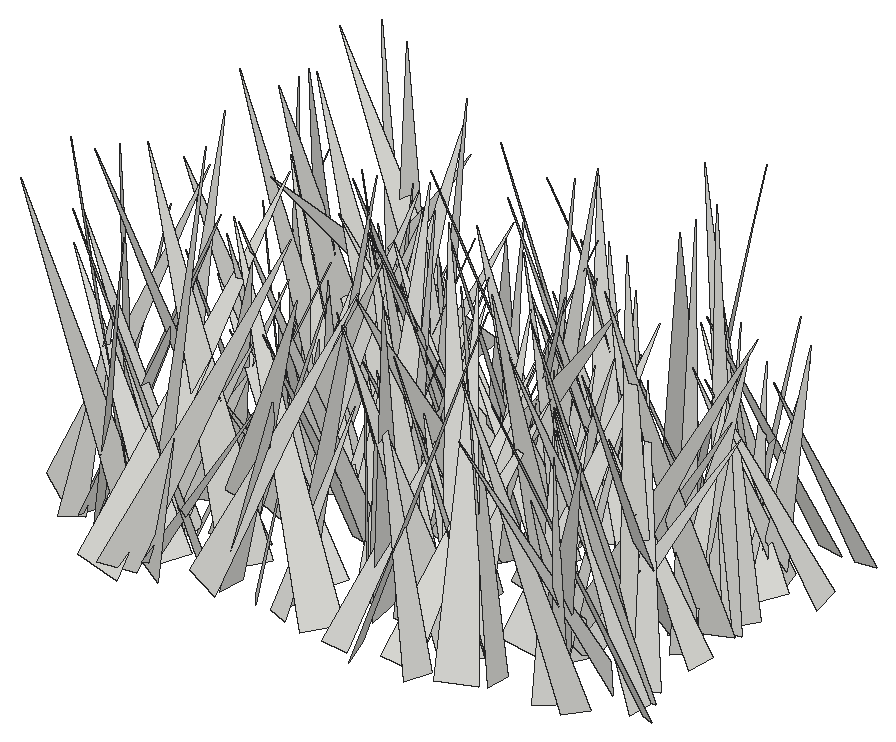
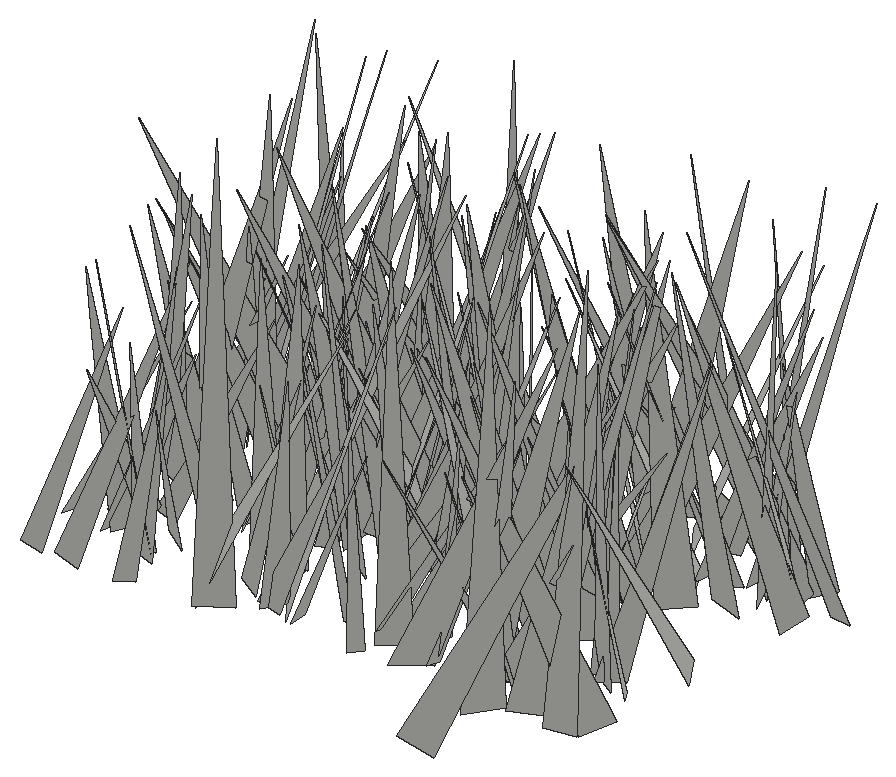
# SketchUp Ruby script. Lengths in inches.
U = 1.inch
M = Sketchup.active_model
def pt(a) = Geom::Point3d.new(a.map { |v| v * U })
def face(e, loops, mat)
  f = e.add_face(loops[0].map { |a| pt(a) })
  loops[1..].each { |l| e.add_face(l.map { |a| pt(a) }).erase! }
  f.material = f.back_material = mat if mat
  f
end
# faces: each face lists its corners as indices into pts; further lists are holes
def faces(e, pts, list, mat = nil) = list.each { |f| face(e, (f[0].is_a?(Array) ? f : [f]).map { |l| l.map { |i| pts[i] } }, mat) }
# xy, xz, yz: faces in a plane at the given z, y or x. An outline is a flat list of corners, or four numbers for a rectangle; further outlines are holes
def ring(l) = l.size == 4 ? [[l[0], l[1]], [l[2], l[1]], [l[2], l[3]], [l[0], l[3]]] : l.each_slice(2).to_a
def flat(e, list, mat, &to3) = list.each { |f| face(e, (f[0].is_a?(Array) ? f : [f]).map { |l| ring(l).map { |u, v| to3.(u, v) } }, mat) }
def xy(e, z, list, mat = nil) = flat(e, list, mat) { |x, y| [x, y, z] }
def xz(e, y, list, mat = nil) = flat(e, list, mat) { |x, z| [x, y, z] }
def yz(e, x, list, mat = nil) = flat(e, list, mat) { |y, z| [x, y, z] }
def lines(e, pts, list) = list.each { |a, b| e.add_line(pt(pts[a]), pt(pts[b])) }
# prism: a flat outline (further loops are holes) pulled along v
def prism(e, loops, v, mat = nil)
  f = face(e, loops, mat); d = Geom::Vector3d.new(v.map { |x| x * U })
  f.pushpull(f.normal.samedirection?(d) ? d.length : -d.length)
end
def box(e, o, s, mat = nil) = prism(e, [[o, [o[0] + s[0], o[1], o[2]], [o[0] + s[0], o[1] + s[1], o[2]], [o[0], o[1] + s[1], o[2]]]], [0, 0, s[2]], mat)
def at(x, y, z, deg = 0) = Geom::Transformation.translation(pt([x, y, z])) * Geom::Transformation.rotation(ORIGIN, Z_AXIS, deg.degrees)
def axes(o, x, y, z) = Geom::Transformation.new([*x, 0, *y, 0, *z, 0, *pt(o).to_a, 1])
def part(name) = M.definitions.add(name)
# library, detail: a bought-in or finely detailed component or shape, given as its bounding box
def library(name, o, s) = part(name).tap { |d| box(d.entities, o, s) }
def detail(e, o, s) = box(e.add_group.entities, o, s)
def put(e, d, t, mat = nil) = e.add_instance(d, t).tap { |i| i.material = mat if mat }
def group(e, t, mat = nil) = e.add_group.tap { |g| g.transformation = t; g.material = mat if mat }.entities
root = M.entities
c1 = part("fur_instance\#9")
p = [[0.8125,0,1.79],[0.67,-0.02,1.48],[0,-0.11,0],[0,0.11,0]]
faces(c1.entities,p,[[0,1,2,3]])
put(root,c1,axes([481.6,86.91,-21.86],[-7.48109,-1.28394,1.71532],[-0.94889,7.57103,1.5286],[1.92105,-1.26035,7.43496]))
put(root,c1,axes([495.89,84.79,-21.86],[-5.54027,1.19429,0.93196],[1.15956,5.61711,-0.30487],[0.97482,0.10593,5.65933]))
put(root,c1,axes([501.27,88.96,-21.86],[-5.37416,-4.85351,0.14678],[-4.51514,5.07548,2.5125],[1.7865,-1.77274,6.79157]))
put(root,c1,axes([480,86.77,-21.66],[6.17791,2.14602,1.95241],[2.61385,-6.11017,-1.55482],[-1.25898,-2.15507,6.35252]))
put(root,c1,axes([485.14,86.22,-21.86],[-5.86461,-3.9483,0.52207],[-3.9663,5.70596,-1.40208],[-0.36068,1.452,6.92942]))
put(root,c1,axes([498.78,88.76,-21.86],[-0.05965,-7.49908,0.31223],[-6.76708,0.1888,3.24163],[3.24657,0.25574,6.76251]))
put(root,c1,axes([493.06,84.84,-21.86],[6.96857,2.87265,0.80723],[2.85827,-7.01507,0.2896],[-0.85676,-0.03815,7.53188]))
put(root,c1,axes([502.04,86.01,-21.66],[-0.7555,-5.85213,2.53673],[-5.87032,-0.36099,-2.58111],[-2.49433,2.62211,5.30623]))
put(root,c1,axes([495.42,87.4375,-21.86],[-6.6748,0.96554,1.83268],[1.43583,6.61336,1.7452],[1.49311,-2.0433,6.51456]))
put(root,c1,axes([483.82,84.82,-21.86],[4.31651,6.80061,2.35568],[7.01576,-4.58865,0.3914],[-1.60519,-1.76799,8.04533]))
put(root,c1,axes([501,86.47,-21.86],[-1.48378,-4.80354,1.85374],[-5.06695,1.70492,0.36217],[0.91449,1.65264,5.01442]))
put(root,c1,axes([492.03,88.03,-21.86],[7.80174,-0.94154,1.76979],[-0.49694,-7.7978,-1.95786],[-1.94209,-1.78708,7.61055]))
put(root,c1,axes([482.92,84.07,-21.66],[6.18283,-3.26103,2.17206],[-3.91127,-5.37775,3.05962],[-0.2327,3.74499,6.28493]))
put(root,c1,axes([486.67,85.82,-21.86],[5.61379,-0.0924,1.25595],[-0.17391,-5.73971,0.3551],[-1.24727,0.38445,5.60331]))
put(root,c1,axes([487.98,85.58,-21.86],[-2.4957,-1.61977,2.11338],[-2.18018,2.90599,-0.34732],[1.52869,1.50005,2.95492]))
put(root,c1,axes([481.2,87.21,-21.86],[-5.20637,-5.83633,2.28098],[-6.06397,5.44004,0.07832],[1.57922,1.64775,7.82067]))
put(root,c1,axes([484.88,88.07,-21.66],[3.43044,-6.71204,0.2285],[-6.5076,-3.25868,1.97581],[1.6598,1.09595,7.27431]))
put(root,c1,axes([483.93,86.05,-21.86],[-4.33384,4.15795,0.46311],[4.09626,4.08164,1.68703],[-0.85069,-1.52868,5.76409]))
put(root,c1,axes([479.18,86.21,-21.86],[3.46953,-2.67132,1.40146],[-2.94376,-3.4648,0.68347],[-0.65905,1.41311,4.3251]))
put(root,c1,axes([486.01,85.03,-21.66],[1.82211,6.46965,0.85286],[6.26515,-1.48669,-2.10749],[1.8253,-1.35544,6.38239]))
put(root,c1,axes([504.28,87.23,-21.66],[-3.99389,-5.07881,0.29207],[-4.86869,3.70838,-2.09153],[-1.47493,1.51142,6.11318]))
put(root,c1,axes([489.29,85.17,-21.86],[1.39427,3.92432,0.17719],[3.92808,-1.39069,-0.10895],[0.04345,-0.20342,4.16322]))
put(root,c1,axes([483.59,85.01,-21.66],[3.8069,0.05751,0.20355],[-0.0416,-3.39391,1.73693],[-0.20739,1.73647,3.38805]))
put(root,c1,axes([491.09,85.42,-21.86],[-3.57557,6.64036,0.56629],[6.42877,3.26724,2.27945],[-1.75672,-1.55901,7.1891]))
put(root,c1,axes([497.24,85.27,-21.86],[-2.95766,6.66869,1.17233],[6.76114,2.97762,0.11972],[0.36439,-1.12067,7.29416]))
put(root,c1,axes([482.18,83.92,-21.86],[0.04279,8.23701,0.26485],[7.98617,0.02394,-2.03491],[2.0346,-0.26721,7.98181]))
put(root,c1,axes([486.22,87.3,-21.86],[-5.61004,5.72169,2.32507],[6.16954,5.3361,1.75473],[0.28367,-2.89906,7.81865]))
put(root,c1,axes([496.71,87.7,-21.86],[-5.00716,-3.11226,0.75462],[-3.18598,4.98296,-0.58898],[0.32424,0.90067,5.86608]))
put(root,c1,axes([498.32,86.27,-21.86],[-7.03444,-1.19576,1.59787],[-1.52444,6.99776,-1.47438],[1.28808,1.75153,6.98136]))
put(root,c1,axes([483.23,87.79,-21.86],[-6.42244,0.41118,0.57395],[0.45958,6.42194,0.54196],[0.53597,-0.57954,6.41273]))
put(root,c1,axes([492.22,84.69,-21.86],[-3.33289,3.23483,0.32122],[2.5841,2.91556,-2.549],[1.97223,1.64647,3.88264]))
put(root,c1,axes([503.16,88.4375,-21.86],[-1.48365,-5.76059,1.44193],[-5.8771,1.21156,-1.20691],[-0.85046,1.67706,5.82486]))
put(root,c1,axes([494.95,84.83,-21.66],[-2.16647,5.60636,0.16983],[5.26617,2.09582,-2.00715],[1.93067,0.57445,5.66535]))
put(root,c1,axes([490.73,88.4375,-21.86],[3.47548,2.68418,2.07766],[3.24177,-3.50628,-0.89294],[-1.00618,-2.02524,4.29959]))
put(root,c1,axes([481.95,87.7,-21.86],[2.31497,4.33574,1.17317],[4.28428,-1.73503,-2.04175],[1.34907,-1.93005,4.47091]))
put(root,c1,axes([503.47,87.96,-21.86],[-5.40823,0.65228,0.52882],[0.69912,5.40686,0.48075],[0.46513,-0.5426,5.42617]))
put(root,c1,axes([491.42,87.84,-21.86],[-2.0645,-2.99831,1.70133],[-3.28642,2.31061,0.08412],[1.04107,1.34824,3.63936]))
put(root,c1,axes([500.58,86.02,-21.86],[-4.64664,1.60589,0.29185],[1.45378,4.47236,-1.46283],[0.74202,1.29401,4.69365]))
put(root,c1,axes([479.47,86.95,-21.86],[6.02676,-0.13267,0.65935],[-0.25057,-5.95995,1.09109],[-0.62414,1.1116,5.92866]))
put(root,c1,axes([499.28,89.35,-21.86],[2.57242,-3.23839,0.522],[-3.12857,-2.6216,-0.84629],[-0.98573,-0.13048,4.04824]))
put(root,c1,axes([480.83,87.65,-21.86],[-6.27895,-2.5321,2.5957],[-2.9165,6.61067,-0.60625],[2.15482,1.56906,6.74309]))
put(root,c1,axes([500.79,91.05,-21.86],[-6.83559,-3.49227,1.59422],[-2.83471,6.78714,2.71329],[2.5888,-1.7893,7.18049]))
put(root,c1,axes([495.28,88.22,-21.86],[-3.28307,2.60382,1.30489],[2.8552,3.26547,0.66758],[0.57484,-1.34832,4.13676]))
put(root,c1,axes([485.5,88.91,-21.86],[-3.35024,-7.10363,1.41562],[-6.97339,2.74138,-2.74705],[-1.95891,2.39017,7.35795]))
put(root,c1,axes([477.58,87.37,-21.86],[3.97232,6.71602,1.21655],[6.692,-3.55551,-2.22255],[1.34242,-2.14887,7.47961]))
put(root,c1,axes([489.41,88.01,-21.86],[-4.10469,4.34568,0.4298],[4.19686,3.76273,2.03626],[-1.20665,-1.6956,5.62024]))
put(root,c1,axes([482.57,87.71,-21.86],[3.62784,4.7769,0.79864],[4.78599,-3.38301,-1.50576],[0.74217,-1.53438,5.80626]))
put(root,c1,axes([485.07,88.8125,-21.86],[5.29628,3.42643,1.15131],[3.61426,-4.98862,-1.7797],[0.0553,-2.11891,6.05175]))
put(root,c1,axes([496.3,86.92,-21.86],[-3.06885,7.2619,1.47031],[7.40414,2.94663,0.90053],[-0.27521,-1.70206,7.83212]))
put(root,c1,axes([482.66,90.24,-21.86],[3.94338,-5.9757,0.15667],[-5.94055,-3.89659,0.90015],[0.66588,0.62564,7.10275]))
put(root,c1,axes([495.98,88.3125,-21.86],[-4.03311,-0.04964,1.55556],[-0.10181,4.31995,-0.1261],[1.55302,0.15428,4.03144]))
put(root,c1,axes([494.17,86.58,-21.66],[-1.05033,5.0969,0.69056],[4.61293,1.24522,-2.17458],[2.27512,-0.17172,4.72788]))
put(root,c1,axes([479.54,87.17,-21.86],[-3.93965,-2.75758,3.63418],[-3.8658,4.56754,-0.72493],[2.42222,2.80458,4.7539]))
put(root,c1,axes([489.33,86.24,-21.86],[-7.34355,0.30763,3.29021],[-0.75169,7.65215,-2.39318],[3.21793,2.48952,6.94946]))
put(root,c1,axes([501.06,90.91,-21.86],[-5.87389,-5.06073,1.31002],[-4.91563,6.01764,1.20596],[1.77871,-0.08191,7.65893]))
put(root,c1,axes([501.11,92.44,-21.66],[-2.73458,-7.67612,0.26637],[-7.34259,2.69559,2.30041],[2.25392,-0.53168,7.81722]))
put(root,c1,axes([478.64,88.625,-21.86],[6.73911,-0.51973,0.37006],[-0.5475,-6.72675,0.52311],[-0.32757,0.55072,6.73884]))
put(root,c1,axes([488.04,89.2,-21.86],[1.13242,-3.28388,1.61058],[-3.44754,-1.52145,-0.67814],[-1.2216,1.24962,3.40681]))
put(root,c1,axes([493.41,88.5625,-21.86],[-2.35431,6.5098,1.98677],[6.74258,1.94391,1.62058],[-0.92858,-2.38982,6.73008]))
put(root,c1,axes([488.35,91.19,-21.86],[-1.09873,-5.30096,0.04279],[-5.29764,1.09638,-0.20521],[-0.19227,0.08352,5.40974]))
put(root,c1,axes([483.35,88.11,-21.86],[5.4364,3.24485,0.19999],[3.25087,-5.4295,-0.27539],[-0.03035,-0.33899,6.32516]))
put(root,c1,axes([492.64,88.92,-21.66],[-4.27144,-3.27285,0.83505],[-3.36103,3.98484,-1.57435],[-0.33515,1.75031,5.14569]))
put(root,c1,axes([486.59,90.29,-21.86],[0.42808,-6.23217,1.75974],[-6.34467,-0.7568,-1.13683],[-1.29687,1.64535,6.14254]))
put(root,c1,axes([493.46,93.06,-21.66],[3.75973,-6.87339,0.18092],[-6.4988,-3.61971,-2.46477],[-2.2454,-1.03249,7.43666]))
put(root,c1,axes([484.69,91.89,-21.66],[-2.93741,-3.09466,0.01129],[-2.71699,2.58635,2.03327],[1.48156,-1.39259,3.75115]))
put(root,c1,axes([490.29,90.08,-21.86],[-2.1287,-6.56011,1.58213],[-6.38568,1.42177,-2.69649],[-2.18201,2.23898,6.34786]))
put(root,c1,axes([497.03,91.3,-21.86],[0.47812,-7.3143,1.47747],[-7.45136,-0.54714,-0.29732],[-0.39895,1.45332,7.32388]))
put(root,c1,axes([484.38,90.89,-21.86],[1.4912,-7.63112,1.5604],[-7.07021,-0.65953,3.53123],[3.26816,2.05513,6.92734]))
put(root,c1,axes([493.02,87.54,-21.86],[3.07038,6.62387,1.59445],[6.28566,-3.42873,2.13997],[-2.62838,-0.46188,6.98022]))
put(root,c1,axes([495.49,88.25,-21.66],[-4.4871,3.83069,1.41429],[3.5666,4.69982,-1.41404],[1.98841,0.2144,5.72789]))
put(root,c1,axes([489.61,90.96,-21.86],[6.19787,3.91116,1.13836],[4.069,-5.84754,-2.06304],[0.19042,-2.34857,7.0324]))
put(root,c1,axes([491.51,90.55,-21.86],[-5.53788,-5.2946,2.37412],[-5.70348,5.57065,-0.88067],[1.06751,2.29618,7.61087]))
put(root,c1,axes([486.34,89.77,-21.66],[3.70498,4.05955,2.96614],[3.93602,-4.63444,1.42637],[-3.1282,-1.02317,5.30776]))
put(root,c1,axes([481.3,89.16,-21.86],[1.99412,7.08431,1.8343],[7.27705,-2.12036,0.27805],[-0.77249,-1.68678,7.35436]))
put(root,c1,axes([503.06,88.7,-21.66],[-0.43332,5.55714,0.38235],[5.39105,0.32188,1.43136],[-1.40165,-0.47995,5.3871]))
put(root,c1,axes([487.06,90.49,-21.66],[-2.6027,-3.00196,0.39616],[-2.70686,2.07255,-2.07851],[-1.35707,1.62343,3.38609]))
put(root,c1,axes([501.82,89.85,-21.86],[-0.81741,7.52572,2.31704],[7.8363,0.54876,0.98214],[-0.77303,-2.39493,7.506]))
put(root,c1,axes([499.68,88,-21.66],[2.78013,5.13783,0.11647],[4.85085,-2.66723,1.86951],[-1.69707,0.79284,5.53456]))
put(root,c1,axes([499.58,89.84,-21.66],[2.70061,4.81345,0.08968],[4.52857,-2.505,-1.92033],[1.63383,-1.01307,5.17446]))
put(root,c1,axes([490.61,89.34,-21.86],[-2.23719,7.0676,1.63885],[7.20712,2.3619,-0.34736],[0.83319,-1.45336,7.40509]))
put(root,c1,axes([497.3,88.7,-21.86],[-1.51128,6.4389,0.97646],[6.11666,1.74753,-2.05657],[2.23592,-0.42848,6.28601]))
put(root,c1,axes([502.22,89.88,-21.86],[-4.46035,-2.40279,1.6408],[-2.85913,4.17643,-1.65628],[0.53948,2.26814,4.788]))
put(root,c1,axes([483.2,92.42,-21.86],[-2.16973,-4.86696,0.63571],[-4.9077,2.16207,-0.19771],[0.07681,0.6613,5.32503]))
put(root,c1,axes([499.56,89.24,-21.86],[-7.36083,-0.13148,0.37404],[-0.23398,7.05478,-2.12469],[0.32007,2.13349,7.04874]))
put(root,c1,axes([497.98,89.49,-21.86],[-2.69846,2.82224,0.09608],[2.72603,2.63813,-0.93001],[0.73688,0.57546,3.79233]))
put(root,c1,axes([503.09,91.73,-21.86],[-4.33776,1.46199,0.55548],[1.55819,4.18055,1.16497],[0.13425,-1.28363,4.42678]))
put(root,c1,axes([492.29,93.375,-21.86],[-5.41835,-3.58553,1.38238],[-3.2455,5.54933,1.6725],[2.0576,-0.68883,6.27832]))
put(root,c1,axes([492.27,94.9,-21.66],[-6.0329,-5.73941,0.68236],[-5.34499,5.91535,2.49841],[2.19943,-1.36753,7.94322]))
put(root,c1,axes([487.82,92.63,-21.66],[5.19096,1.17327,0.15724],[1.14991,-4.82989,-1.92283],[0.28108,-1.90867,4.96239]))
put(root,c1,axes([498.68,90.24,-21.66],[6.56364,-3.25708,1.01889],[-3.38805,-5.95385,2.79299],[0.40967,2.94467,6.77415]))
put(root,c1,axes([494.46,91.16,-21.86],[-3.43885,-1.25141,0.28396],[-1.28081,3.29756,-0.97876],[-0.07859,1.01608,3.52615]))
put(root,c1,axes([483.93,91.53,-21.86],[3.27603,2.91205,0.73309],[2.99826,-3.11162,-1.03833],[0.1671,-1.26001,4.25844]))
put(root,c1,axes([494.68,92.12,-21.86],[0.8957,-3.44027,0.95903],[-3.38159,-0.49886,1.36875],[1.14894,1.21373,3.28089]))
put(root,c1,axes([492,93.84,-21.66],[-3.24466,-1.65637,0.06319],[-1.44148,2.88818,1.68993],[0.81834,-1.47993,3.2273]))
put(root,c1,axes([502.38,93.41,-21.66],[0.14854,-7.36709,1.66817],[-7.40985,-0.46607,-1.39849],[-1.46661,1.60862,7.23466]))
put(root,c1,axes([492.3,92.89,-21.66],[1.15805,-3.96128,0.43832],[-3.70743,-0.90324,1.63219],[1.46246,0.84697,3.79062]))
put(root,c1,axes([495.09,93.5,-21.86],[-3.74984,-6.28849,1.24601],[-6.40364,3.74219,-0.38514],[0.30173,1.26879,7.3115]))
put(root,c1,axes([496.51,92.26,-21.86],[-4.30239,2.31555,0.00735],[2.25428,4.18495,1.12996],[-0.52922,-0.99839,4.75348]))
put(root,c1,axes([490.18,93.12,-21.86],[4.31656,-7.06636,0.27005],[-6.24466,-3.6606,4.0303],[3.31821,2.3034,7.23345]))
put(root,c1,axes([498.3,92.22,-21.86],[4.90095,-2.69617,0.00541],[-2.57457,-4.67657,1.67032],[0.80058,1.46597,5.33842]))
put(root,c1,axes([495.54,92.51,-21.86],[2.79577,3.11606,1.7882],[3.42019,-3.00212,-0.11591],[-1.09992,-1.41467,4.18482]))
put(root,c1,axes([492.37,91.15,-21.86],[3.37937,2.22818,0.23171],[2.15143,-3.34494,0.78826],[-0.62436,0.53406,3.97033]))
put(root,c1,axes([490.51,90.8,-21.86],[-0.0626,5.05917,0.30688],[5.04763,0.09003,-0.45456],[0.45914,-0.29998,5.03909]))
put(root,c1,axes([492.65,93.74,-21.86],[6.84395,0.46131,0.76105],[0.6015,-6.74756,-1.31919],[-0.65589,-1.3745,6.73144]))
put(root,c1,axes([489.65,93.23,-21.86],[5.36084,-0.19835,3.29768],[0.06393,-6.27827,-0.48156],[-3.30302,-0.44345,5.34285]))
put(root,c1,axes([483.56,93.9,-21.86],[1.83451,-3.56347,0.05806],[-3.52397,-1.80394,0.62811],[0.53227,0.33851,3.95843]))
put(root,c1,axes([482.54,94.04,-21.86],[-0.97115,-4.17934,0.95629],[-4.09852,1.19278,1.05068],[1.25838,0.65947,4.16006]))
put(root,c1,axes([495.01,93.85,-21.66],[4.68158,-4.31782,3.21331],[-4.18207,-5.59908,-1.43065],[-3.3881,0.94493,6.20597]))
put(root,c1,axes([494.79,94.77,-21.66],[4.08531,-1.79648,1.28746],[-1.24322,-4.1049,-1.78292],[-1.82737,-1.22355,4.09124]))
put(root,c1,axes([491.63,94.3,-21.86],[-2.75065,-6.97463,1.22589],[-6.99898,2.47729,-1.60986],[-1.07823,1.71227,7.32256]))
put(root,c1,axes([489.38,94.33,-21.86],[-0.13278,-3.81265,0.23397],[-3.74221,0.08288,-0.77308],[-0.76609,0.25594,3.73581]))
put(root,c1,axes([494.83,93.55,-21.86],[4.10289,-2.86128,0.97197],[-3.01034,-4.01302,0.89377],[-0.2636,1.29386,4.92156]))
put(root,c1,axes([496.3125,94.58,-21.86],[-5.74525,-5.95088,0.61636],[-5.93253,5.55629,-1.65334],[-0.77329,1.58601,8.10478]))
put(root,c1,axes([484.39,92.54,-21.66],[0.24671,6.36494,1.6516],[6.30189,0.24313,-1.87833],[1.87786,-1.65213,6.08648]))
put(root,c1,axes([496.76,94.37,-21.86],[-3.60372,1.36671,1.25031],[1.68423,3.55609,0.96723],[0.77106,-1.37995,3.73084]))
put(root,c1,axes([491.88,93.93,-21.86],[-3.57331,4.48467,0.98446],[4.4978,3.16833,1.89248],[-0.92266,-1.92337,5.41289]))
put(root,c1,axes([481.65,95.95,-21.66],[4.12034,-0.14152,0.59374],[0.17297,-3.61498,-2.06197],[-0.58535,-2.06437,3.57009]))
put(root,c1,axes([481.18,95.8,-21.86],[5.01755,-2.86523,2.69296],[-2.1597,-5.65647,-1.99435],[-3.28592,-0.6574,5.42291]))
put(root,c1,axes([498.92,93.48,-21.86],[-1.92431,3.57441,0.40694],[3.46774,1.72017,1.28872],[-0.95749,-0.95373,3.84949]))
put(root,c1,axes([501.4,92.69,-21.86],[-0.62067,4.74172,0.56344],[4.77083,0.63973,-0.12835],[0.20124,-0.5417,4.78044]))
put(root,c1,axes([492.55,93.4,-21.86],[1.055,3.81063,1.04337],[3.83467,-1.24762,0.6792],[-0.95124,-0.80317,3.89521]))
put(root,c1,axes([487.48,92.42,-21.66],[-4.32625,3.6169,1.13686],[3.35652,4.45591,-1.40339],[1.76301,0.39209,5.46158]))
put(root,c1,axes([491.28,92.08,-21.86],[5.73522,3.47371,0.17785],[3.39582,-5.66618,1.16354],[-0.75282,0.90483,6.60345]))
put(root,c1,axes([483.65,92.77,-21.86],[-0.33332,4.6985,0.41104],[4.65173,0.39553,-0.74898],[0.77866,-0.35159,4.65038]))
put(root,c1,axes([498.14,94.76,-21.86],[3.40491,-1.73217,0.1961],[-1.74293,-3.39081,0.31125],[-0.03288,0.3664,3.80749]))
put(root,c1,axes([497.35,95.47,-21.86],[-6.81995,-3.62088,0.84533],[-3.65528,6.85252,-0.13797],[0.68141,0.51893,7.72033]))
put(root,c1,axes([493.19,92.6,-21.66],[-6.05732,0.47074,1.68041],[-0.07648,5.99257,-1.95441],[1.74342,1.89841,5.75265]))
put(root,c1,axes([498.39,94.84,-21.86],[-4.80301,-2.64529,0.12183],[-2.62964,4.73476,-0.865],[-0.31202,0.81591,5.41463]))
put(root,c1,axes([484.19,95.35,-21.86],[-7.83608,-0.63477,1.59162],[-0.4911,7.96997,0.76075],[1.64165,-0.64574,7.82485]))
put(root,c1,axes([500.04,94.45,-21.86],[-1.7832,4.7887,2.83203],[5.02838,2.65983,-1.33139],[2.38064,-2.03113,4.93345]))
put(root,c1,axes([489.93,92.92,-21.66],[3.45024,7.01244,2.07893],[6.95776,-3.8555,1.45774],[-2.25516,-1.1667,7.67811]))
put(root,c1,axes([502.15,91.92,-21.86],[-7.67594,0.43258,1.18162],[-0.05572,7.18028,-2.99063],[1.25708,2.9597,7.0826]))
put(root,c1,axes([495.43,93.18,-21.86],[0.25291,3.93977,0.05992],[3.89833,-0.25892,0.57035],[-0.57304,-0.02262,3.90646]))
put(root,c1,axes([500.79,96.28,-21.86],[-0.19761,-4.29399,0.26182],[-4.09062,0.10641,-1.34218],[-1.33181,0.31028,4.08362]))
put(root,c1,axes([482.98,96.15,-21.86],[0.8236,-4.35079,0.44599],[-4.32851,-0.74586,0.71716],[0.62636,0.56649,4.3696]))
put(root,c1,axes([485.59,93.5,-21.86],[-1.50811,5.89701,0.63499],[5.61901,1.21081,2.10069],[-1.89858,-1.1007,5.71281]))
put(root,c1,axes([489.25,95.24,-21.86],[-4.02078,2.93374,1.78068],[3.22926,4.16274,0.43339],[1.1617,-1.41743,4.95839]))
put(root,c1,axes([485.93,95.59,-21.86],[3.66443,-1.25509,0.51627],[-1.25966,-3.69872,-0.05095],[-0.50503,0.11865,3.87307]))
put(root,c1,axes([494.21,93.52,-21.66],[-6.74927,1.80081,2.69667],[1.18797,7.16726,-1.81295],[3.01723,1.2063,6.74602]))
put(root,c1,axes([486.32,93.76,-21.86],[-1.25446,7.26591,1.58891],[7.27727,1.53186,-1.25954],[1.53602,-1.32352,7.26503]))
put(root,c1,axes([496.72,95.68,-21.86],[4.30224,-3.16543,2.15858],[-3.43037,-4.62804,0.05027],[-1.70646,1.32286,5.34104]))
put(root,c1,axes([489.27,96.91,-21.86],[-5.99784,0.36822,0.31916],[0.44096,5.77868,1.61988],[0.20737,-1.63795,5.78668]))
put(root,c1,axes([502.34,94.03,-21.86],[0.70044,7.59304,1.85976],[7.56257,-1.13109,1.76971],[-1.98005,-1.63401,7.41708]))
put(root,c1,axes([485.41,94.72,-21.86],[3.56009,0.21869,0.65734],[0.01468,-3.46445,1.07311],[-0.69261,1.05069,3.40155]))
put(root,c1,axes([493.25,94.92,-21.86],[3.25616,5.95918,2.11371],[6.15078,-3.5363,0.49462],[-1.46542,-1.60155,6.77272]))
put(root,c1,axes([480.08,96.29,-21.86],[3.15545,2.01724,0.79775],[2.15051,-3.09372,-0.68323],[-0.2846,-1.01105,3.6823]))
put(root,c1,axes([479.14,93.78,-21.66],[4.7893,3.01055,0.30481],[2.77693,-4.59952,1.79634],[-1.20208,1.36921,5.36414]))
put(root,c1,axes([485.99,96.61,-21.86],[-6.02527,4.37662,1.94606],[4.73834,5.90349,1.39383],[0.70004,-2.28907,7.31546]))
put(root,c1,axes([488.75,98.49,-21.86],[1.84605,-6.6162,0.27609],[-6.51912,-1.76548,1.28157],[1.16252,0.60597,6.74831]))
put(root,c1,axes([484.09,98.2,-21.86],[6.81977,1.54998,0.06465],[1.44583,-6.24479,-2.79788],[0.56233,-2.74155,6.40965]))
put(root,c1,axes([494.41,96.6,-21.86],[3.27913,1.40298,0.59687],[1.4938,-3.23974,-0.59158],[-0.30522,-0.78299,3.51725]))
put(root,c1,axes([481.4,95.95,-21.86],[3.04497,5.63186,2.55497],[5.93211,-3.46487,0.56775],[-1.7481,-1.94792,6.3771]))
put(root,c1,axes([489.45,98.14,-21.66],[-4.59032,-0.23962,0.17171],[-0.16134,4.28449,1.66587],[0.24672,-1.65642,4.28408]))
put(root,c1,axes([502.66,94.55,-21.66],[-8.1921,1.36867,0.61461],[1.20152,8.02801,-1.8625],[0.89853,1.74336,8.09413]))
put(root,c1,axes([503.6875,98,-21.86],[-4.90231,-0.23018,0.15933],[-0.18525,4.76264,1.18065],[0.20988,-1.17272,4.76358]))
put(root,c1,axes([501.85,98.21,-21.86],[-4.7933,-0.97536,0.74224],[-0.77682,4.73507,1.20565],[0.94805,-1.05153,4.74061]))
put(root,c1,axes([487.96,96.71,-21.86],[-4.49863,-0.46507,1.40367],[-0.60193,4.68178,-0.37796],[1.35065,0.53749,4.50678]))
put(root,c1,axes([482.48,97.14,-21.66],[0.05129,-4.93553,2.34933],[-4.99892,0.90807,2.01684],[2.21125,2.16734,4.50493]))
put(root,c1,axes([481.99,99.34,-21.86],[5.20163,-5.29224,1.8402],[-4.95757,-5.51713,-1.85336],[-2.61089,-0.0677,7.18539]))
put(root,c1,axes([486.84,98.66,-21.86],[-4.25051,-1.02119,0.70994],[-0.79222,4.17184,1.25768],[0.95876,-1.08007,4.18663]))
put(root,c1,axes([480.32,99.7,-21.86],[-1.25565,-8.18969,1.33935],[-8.04493,1.53362,1.83538],[2.03567,1.00923,8.07955]))
put(root,c1,axes([495.2,96.46,-21.86],[-2.95923,6.17255,1.7602],[6.41346,2.92118,0.53848],[0.25723,-1.82266,6.82403]))
put(root,c1,axes([495.2,100.5625,-21.66],[1.43301,-8.2393,0.15598],[-8.02359,-1.35888,1.93375],[1.87948,0.48092,8.13635]))
put(root,c1,axes([495.32,98.43,-21.86],[-2.87551,-4.98025,1.4124],[-5.17006,2.84441,-0.49611],[0.26119,1.47404,5.72934]))
put(root,c1,axes([490.94,98.26,-21.86],[3.06956,3.90435,1.71137],[4.25532,-2.68017,-1.51785],[0.25498,-2.27325,4.72887]))
put(root,c1,axes([502.1,97.05,-21.86],[-3.00277,4.1066,0.06153],[3.92812,2.84936,1.52829],[-1.19912,-0.94951,4.85234]))
put(root,c1,axes([501.38,97.77,-21.86],[4.20018,-2.603,1.54886],[-2.85846,-4.28223,0.55487],[-1.0019,1.30501,4.91012]))
put(root,c1,axes([484.49,97.3,-21.86],[4.52412,1.43506,1.852],[1.32361,-4.8885,0.5546],[-1.93323,0.01133,4.71375]))
put(root,c1,axes([484.22,98.03,-21.86],[-2.52559,2.65872,0.46687],[2.62617,2.27215,1.26725],[-0.62447,-1.19747,3.44114]))
put(root,c1,axes([487.69,97.17,-21.86],[-3.44021,1.49763,0.22694],[1.46636,3.43395,-0.43273],[0.37973,0.30751,3.72702]))
put(root,c1,axes([489.3,99.95,-21.66],[-0.15941,-4.26775,0.08772],[-3.87813,0.18147,1.78158],[1.78369,0.01316,3.88138]))
put(root,c1,axes([499.67,99.02,-21.86],[-1.75963,-5.21212,1.71135],[-5.46295,1.82898,-0.04671],[0.50104,1.63703,5.50093]))
put(root,c1,axes([493.37,98.75,-21.86],[-5.74367,-4.09689,1.01684],[-4.21686,5.6466,-1.0688],[0.19121,1.46278,6.97366]))
put(root,c1,axes([501.24,96.52,-21.86],[-3.77654,1.99621,0.89861],[1.50689,3.67022,-1.82025],[1.58796,1.26459,3.86442]))
put(root,c1,axes([479.4,98.71,-21.86],[3.63581,-6.29578,1.08718],[-5.74464,-2.67402,3.72648],[2.79605,2.69271,6.24254]))
put(root,c1,axes([482.97,98.77,-21.86],[2.90459,3.11145,0.76807],[3.13189,-2.53582,-1.57117],[0.67994,-1.61126,3.9559]))
put(root,c1,axes([499.43,98.86,-21.86],[4.01593,3.70117,1.52807],[3.99587,-3.8439,-1.19115],[-0.25835,-1.92018,5.32987]))
put(root,c1,axes([501.55,100.91,-21.86],[-1.38983,-5.84462,0.0201],[-5.82782,1.38425,-0.46046],[-0.44334,0.12603,5.98992]))
put(root,c1,axes([499.84,98.67,-21.86],[0.95056,-3.70171,1.6828],[-4.06505,-0.90725,0.30052],[-0.09921,1.70654,3.80998]))
put(root,c1,axes([485.76,96.73,-21.66],[-7.72963,0.57294,0.92033],[0.30078,7.49944,-2.14251],[1.04153,2.08628,7.44883]))
put(root,c1,axes([484.56,97.32,-21.86],[1.65691,4.63189,0.02775],[4.518,-1.60961,-1.09423],[1.0212,-0.39403,4.79608]))
put(root,c1,axes([492.55,99.16,-21.86],[-3.97846,-0.22397,0.26493],[-0.21326,3.98441,0.16592],[0.27363,-0.15114,3.9813]))
put(root,c1,axes([493.87,99.12,-21.86],[-1.39517,3.65073,1.37856],[3.73252,0.82124,1.60268],[-1.13865,-1.78115,3.56451]))
put(root,c1,axes([497.92,97.06,-21.66],[6.4621,3.38539,1.99868],[3.00841,-6.73382,1.67909],[-2.53082,0.63956,7.09931]))
put(root,c1,axes([487.4,99.21,-21.86],[-7.15301,3.97515,0.71331],[4.02795,6.91641,1.848],[-0.2937,-1.95899,7.97197]))
put(root,c1,axes([483.41,103.96,-21.66],[5.32765,-5.22538,0.29084],[-4.03169,-4.36253,-4.52625],[-3.33686,-3.07194,5.93309]))
put(root,c1,axes([503.12,100.92,-21.86],[-0.25255,-4.7231,0.0991],[-4.68784,0.23828,-0.59045],[-0.58449,0.12972,4.69284]))
put(root,c1,axes([499.47,97.4,-21.86],[1.37607,4.21587,0.41156],[3.82506,-1.42264,1.78368],[-1.81985,0.19763,4.06025]))
put(root,c1,axes([496.56,99.95,-21.86],[-5.23491,-4.53939,0.15815],[-4.43832,5.06084,-1.65066],[-0.96564,1.34804,6.72946]))
put(root,c1,axes([493.78,98.92,-21.86],[-4.02288,2.74208,1.38872],[2.85785,4.17888,0.02734],[1.13147,-0.80565,4.86845]))
put(root,c1,axes([499.01,100.81,-21.86],[3.89618,-1.88557,1.1779],[-1.51971,-3.99347,-1.36592],[-1.62275,-0.78732,4.1073]))
put(root,c1,axes([483.33,100.23,-21.86],[6.49174,-3.69034,2.54193],[-3.75607,-6.92147,-0.45599],[-2.44375,0.83512,7.45341]))
